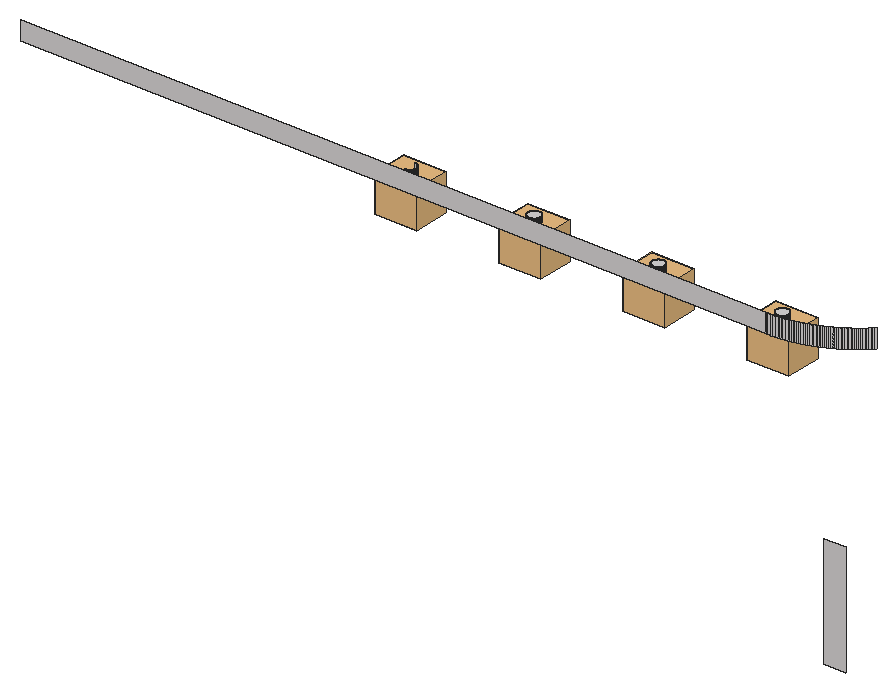
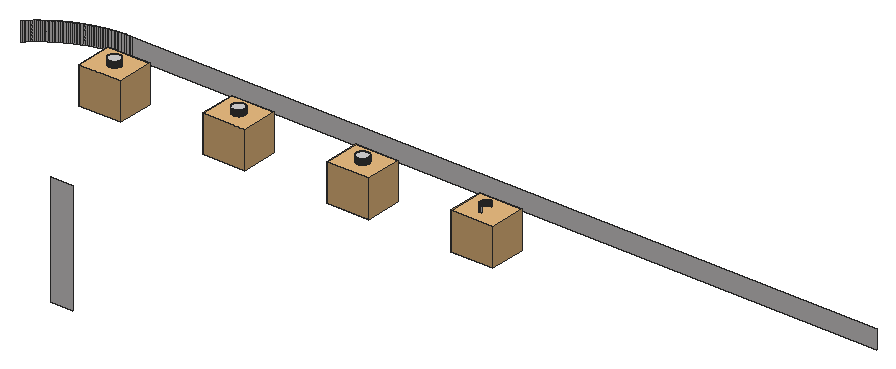
# SketchUp Ruby script. Lengths in inches.
U = 1.inch
M = Sketchup.active_model
def pt(a) = Geom::Point3d.new(a.map { |v| v * U })
def face(e, loops, mat)
  f = e.add_face(loops[0].map { |a| pt(a) })
  loops[1..].each { |l| e.add_face(l.map { |a| pt(a) }).erase! }
  f.material = f.back_material = mat if mat
  f
end
# faces: each face lists its corners as indices into pts; further lists are holes
def faces(e, pts, list, mat = nil) = list.each { |f| face(e, (f[0].is_a?(Array) ? f : [f]).map { |l| l.map { |i| pts[i] } }, mat) }
# xy, xz, yz: faces in a plane at the given z, y or x. An outline is a flat list of corners, or four numbers for a rectangle; further outlines are holes
def ring(l) = l.size == 4 ? [[l[0], l[1]], [l[2], l[1]], [l[2], l[3]], [l[0], l[3]]] : l.each_slice(2).to_a
def flat(e, list, mat, &to3) = list.each { |f| face(e, (f[0].is_a?(Array) ? f : [f]).map { |l| ring(l).map { |u, v| to3.(u, v) } }, mat) }
def xy(e, z, list, mat = nil) = flat(e, list, mat) { |x, y| [x, y, z] }
def xz(e, y, list, mat = nil) = flat(e, list, mat) { |x, z| [x, y, z] }
def yz(e, x, list, mat = nil) = flat(e, list, mat) { |y, z| [x, y, z] }
def lines(e, pts, list) = list.each { |a, b| e.add_line(pt(pts[a]), pt(pts[b])) }
# prism: a flat outline (further loops are holes) pulled along v
def prism(e, loops, v, mat = nil)
  f = face(e, loops, mat); d = Geom::Vector3d.new(v.map { |x| x * U })
  f.pushpull(f.normal.samedirection?(d) ? d.length : -d.length)
end
def box(e, o, s, mat = nil) = prism(e, [[o, [o[0] + s[0], o[1], o[2]], [o[0] + s[0], o[1] + s[1], o[2]], [o[0], o[1] + s[1], o[2]]]], [0, 0, s[2]], mat)
def at(x, y, z, deg = 0) = Geom::Transformation.translation(pt([x, y, z])) * Geom::Transformation.rotation(ORIGIN, Z_AXIS, deg.degrees)
def axes(o, x, y, z) = Geom::Transformation.new([*x, 0, *y, 0, *z, 0, *pt(o).to_a, 1])
def part(name) = M.definitions.add(name)
# library, detail: a bought-in or finely detailed component or shape, given as its bounding box
def library(name, o, s) = part(name).tap { |d| box(d.entities, o, s) }
def detail(e, o, s) = box(e.add_group.entities, o, s)
def put(e, d, t, mat = nil) = e.add_instance(d, t).tap { |i| i.material = mat if mat }
def group(e, t, mat = nil) = e.add_group.tap { |g| g.transformation = t; g.material = mat if mat }.entities
root = M.entities
M.materials.add("[Quartz Light Brown]").color = [215, 212, 212]
c1 = library("3",[-5.26,-4.28,-11.86],[13.52,11.56,11.86])
xy(root,483,[[384.27,287.7,384.11,287.71,383.81,287.77,383.66,287.82,383.51,287.88,383.37,287.95,383.24,288.03,383.11,288.12,382.99,288.22,382.875,288.33,382.77,288.45,382.68,288.58,382.6,288.71,382.52,288.85,382.46,288.99,382.41,289.14,382.375,289.29,382.35,289.45,382.34,289.61,382.33,289.76,382.37,290.08,382.4,290.23,382.45,290.38,382.51,290.52,382.58,290.66,382.66,290.8,382.75,290.93,382.85,291.05,382.96,291.16,383.08,291.26,383.21,291.35,383.34,291.4375,383.48,291.51,383.625,291.57,383.77,291.62,383.93,291.66,384.08,291.69,384.24,291.7,384.4,291.7,384.55,291.6875,384.71,291.67,384.86,291.63,385.01,291.58,385.16,291.52,385.3,291.45,385.43,291.37,385.56,291.28,385.68,291.18,385.79,291.07,385.99,290.83,386.07,290.69,386.14,290.55,386.2,290.41,386.25,290.26,386.29,290.11,386.32,289.95,386.33,289.8,386.33,289.64,386.32,289.48,386.3,289.33,386.26,289.17,386.22,289.02,386.16,288.88,386.09,288.74,386.01,288.6,385.91,288.48,385.8125,288.36,385.7,288.24,385.58,288.14,385.46,288.05,385.32,287.96,385.19,287.89,385.04,287.83,384.89,287.78,384.74,287.74,384.58,287.72,384.43,287.7],[424.1,287.7,423.95,287.71,423.79,287.74,423.64,287.77,423.49,287.82,423.34,287.88,423.2,287.95,423.07,288.03,422.94,288.12,422.82,288.22,422.71,288.33,422.61,288.45,422.51,288.58,422.43,288.71,422.36,288.85,422.3,288.99,422.25,289.14,422.21,289.29,422.18,289.45,422.17,289.61,422.17,289.76,422.18,289.92,422.2,290.08,422.28,290.38,422.34,290.52,422.41,290.66,422.49,290.8,422.59,290.93,422.6875,291.05,422.8,291.16,422.92,291.26,423.04,291.35,423.18,291.4375,423.31,291.51,423.46,291.57,423.61,291.62,423.76,291.66,423.92,291.69,424.07,291.7,424.23,291.7,424.39,291.6875,424.54,291.67,424.69,291.63,424.84,291.58,424.99,291.52,425.13,291.45,425.26,291.37,425.39,291.28,425.51,291.18,425.625,291.07,425.73,290.95,425.82,290.83,425.98,290.55,426.04,290.41,426.09,290.26,426.125,290.11,426.15,289.95,426.16,289.8,426.17,289.64,426.15,289.48,426.13,289.33,426.1,289.17,426.05,289.02,425.99,288.88,425.92,288.74,425.84,288.6,425.75,288.48,425.65,288.36,425.54,288.24,425.42,288.14,425.16,287.96,425.02,287.89,424.875,287.83,424.73,287.78,424.57,287.74,424.42,287.72,424.26,287.7],[463.9375,287.7,463.78,287.71,463.47,287.77,463.32,287.82,463.18,287.88,463.04,287.95,462.9,288.03,462.77,288.12,462.65,288.22,462.54,288.33,462.44,288.45,462.26,288.71,462.19,288.85,462.13,288.99,462.08,289.14,462.04,289.29,462,289.61,462,289.76,462.01,289.92,462.04,290.08,462.07,290.23,462.12,290.38,462.18,290.52,462.25,290.66,462.33,290.8,462.42,290.93,462.52,291.05,462.63,291.16,462.75,291.26,462.875,291.35,463.01,291.4375,463.15,291.51,463.29,291.57,463.44,291.62,463.59,291.66,463.75,291.69,463.91,291.7,464.0625,291.7,464.22,291.6875,464.375,291.67,464.53,291.63,464.68,291.58,464.82,291.52,464.96,291.45,465.1,291.37,465.23,291.28,465.35,291.18,465.46,291.07,465.56,290.95,465.65,290.83,465.74,290.69,465.81,290.55,465.87,290.41,465.92,290.26,465.96,290.11,465.98,289.95,466,289.8,466,289.64,465.99,289.48,465.96,289.33,465.93,289.17,465.88,289.02,465.82,288.88,465.75,288.74,465.67,288.6,465.58,288.48,465.48,288.36,465.37,288.24,465.25,288.14,465.125,288.05,464.99,287.96,464.85,287.89,464.71,287.83,464.56,287.78,464.41,287.74,464.09,287.7]],"[Quartz Light Brown]")
xz(root,276.5,[[488,396,495,432]],"[Quartz Light Brown]")
xz(root,282.7,[[225,480,464,486],[464,480,464.5,486]],"[Quartz Light Brown]")
xz(root,287.7,[[344.4375,480,344.59,483],[384.27,480,384.43,483],[424.1,480,424.26,483],[463.9375,480,464.09,483]],"[Quartz Light Brown]")
xz(root,291.7,[[384.24,480,384.4,483],[424.07,480,424.23,483],[463.91,480,464.0625,483]],"[Quartz Light Brown]")
yz(root,346.5,[[289.64,480,289.8,483]],"[Quartz Light Brown]")
yz(root,386.33,[[289.64,480,289.8,483]],"[Quartz Light Brown]")
yz(root,422.17,[[289.61,480,289.76,483]],"[Quartz Light Brown]")
yz(root,462,[[289.61,480,289.76,483]],"[Quartz Light Brown]")
yz(root,466,[[289.64,480,289.8,483]],"[Quartz Light Brown]")
p = [[464.5,282.7,480],[464.99,282.71,480],[464.99,282.71,486],[464.5,282.7,486],[465.49,282.73,480],[465.49,282.73,486],
  [465.99,282.75,480],[465.99,282.75,486],[466.49,282.78,480],[466.49,282.78,486],[466.98,282.82,480],[466.98,282.82,486],
  [467.48,282.86,480],[467.48,282.86,486],[467.97,282.91,480],[467.97,282.91,486],[468.47,282.96,480],[468.47,282.96,486],
  [468.96,283.03,480],[468.96,283.03,486],[469.45,283.09,480],[469.45,283.09,486],[469.94,283.17,480],[469.94,283.17,486],
  [470.44,283.25,480],[470.44,283.25,486],[470.92,283.34,480],[470.92,283.34,486],[471.41,283.43,480],[471.41,283.43,486],
  [471.9,283.53,480],[471.9,283.53,486],[472.39,283.64,480],[472.39,283.64,486],[472.87,283.75,480],[472.87,283.75,486],
  [473.35,283.87,480],[473.35,283.87,486],[473.84,284,480],[473.84,284,486],[474.31,284.13,480],[474.31,284.13,486],
  [474.79,284.27,480],[474.79,284.27,486],[475.27,284.41,480],[475.27,284.41,486],[475.74,284.5625,480],[475.74,284.5625,486],
  [476.21,284.72,480],[476.21,284.72,486],[476.68,284.88,480],[476.68,284.88,486],[477.15,285.05,480],[477.15,285.05,486],
  [477.62,285.22,480],[477.62,285.22,486],[478.08,285.41,480],[478.08,285.41,486],[478.54,285.59,480],[478.54,285.59,486],
  [479,285.79,480],[479,285.79,486],[479.46,285.99,480],[479.46,285.99,486],[479.91,286.19,480],[479.91,286.19,486],
  [480.36,286.4,480],[480.36,286.4,486],[480.81,286.62,480],[480.81,286.62,486],[481.25,286.84,480],[481.25,286.84,486],
  [481.69,287.07,480],[481.69,287.07,486],[482.13,287.31,480],[482.13,287.31,486],[482.57,287.55,480],[482.57,287.55,486],
  [483,287.79,480],[483,287.79,486],[344.75,287.72,480],[344.59,287.7,480],[344.59,287.7,483],[344.75,287.72,483],
  [344.91,287.74,480],[344.91,287.74,483],[345.06,287.78,480],[345.06,287.78,483],[383.96,287.74,480],[383.81,287.77,480],
  [383.81,287.77,483],[383.96,287.74,483],[384.11,287.71,480],[384.11,287.71,483],[384.27,287.7,480],[384.27,287.7,483],
  [384.58,287.72,480],[384.43,287.7,480],[384.43,287.7,483],[384.58,287.72,483],[384.74,287.74,480],[384.74,287.74,483],
  [384.89,287.78,480],[384.89,287.78,483],[423.79,287.74,480],[423.64,287.77,480],[423.64,287.77,483],[423.79,287.74,483],
  [423.95,287.71,480],[423.95,287.71,483],[424.1,287.7,480],[424.1,287.7,483],[424.42,287.72,480],[424.26,287.7,480],
  [424.26,287.7,483],[424.42,287.72,483],[424.57,287.74,480],[424.57,287.74,483],[424.73,287.78,480],[424.73,287.78,483],
  [463.625,287.74,480],[463.47,287.77,480],[463.47,287.77,483],[463.625,287.74,483],[463.78,287.71,480],[463.78,287.71,483],
  [463.9375,287.7,480],[463.9375,287.7,483],[464.25,287.72,480],[464.09,287.7,480],[464.09,287.7,483],[464.25,287.72,483],
  [464.41,287.74,480],[464.41,287.74,483],[464.56,287.78,480],[464.56,287.78,483],[345.21,287.83,480],[345.21,287.83,483],
  [345.35,287.89,480],[345.35,287.89,483],[383.66,287.82,480],[383.51,287.88,480],[383.51,287.88,483],[383.66,287.82,483],
  [385.04,287.83,480],[385.04,287.83,483],[385.19,287.89,480],[385.19,287.89,483],[423.49,287.82,480],[423.34,287.88,480],
  [423.34,287.88,483],[423.49,287.82,483],[424.875,287.83,480],[424.875,287.83,483],[425.02,287.89,480],[425.02,287.89,483],
  [463.32,287.82,480],[463.18,287.88,480],[463.18,287.88,483],[463.32,287.82,483],[464.71,287.83,480],[464.71,287.83,483],
  [464.85,287.89,480],[464.85,287.89,483],[483.43,288.04,480],[483.43,288.04,486],[345.49,287.96,480],[345.49,287.96,483],
  [383.37,287.95,480],[383.24,288.03,480],[383.24,288.03,483],[383.37,287.95,483],[385.32,287.96,480],[385.32,287.96,483],
  [423.2,287.95,480],[423.07,288.03,480],[423.07,288.03,483],[423.2,287.95,483],[425.16,287.96,480],[425.16,287.96,483],
  [463.04,287.95,480],[462.9,288.03,480],[462.9,288.03,483],[463.04,287.95,483],[464.99,287.96,480],[464.99,287.96,483],
  [345.625,288.05,480],[345.625,288.05,483],[345.75,288.14,480],[345.75,288.14,483],[383.11,288.12,480],[383.11,288.12,483],
  [385.46,288.05,480],[385.46,288.05,483],[385.58,288.14,480],[385.58,288.14,483],[422.94,288.12,480],[422.94,288.12,483],
  [425.29,288.05,480],[425.29,288.05,483],[425.42,288.14,480],[425.42,288.14,483],[462.77,288.12,480],[462.77,288.12,483],
  [465.125,288.05,480],[465.125,288.05,483],[465.25,288.14,480],[465.25,288.14,483],[483.85,288.3,480],[483.85,288.3,486],
  [345.87,288.24,480],[345.87,288.24,483],[382.99,288.22,480],[382.99,288.22,483],[385.7,288.24,480],[385.7,288.24,483],
  [422.82,288.22,480],[422.82,288.22,483],[425.54,288.24,480],[425.54,288.24,483],[462.65,288.22,480],[462.65,288.22,483],
  [465.37,288.24,480],[465.37,288.24,483],[345.98,288.36,480],[345.98,288.36,483],[382.875,288.33,480],[382.875,288.33,483],
  [385.8125,288.36,480],[385.8125,288.36,483],[422.71,288.33,480],[422.71,288.33,483],[425.65,288.36,480],[425.65,288.36,483],
  [462.54,288.33,480],[462.54,288.33,483],[465.48,288.36,480],[465.48,288.36,483],[382.77,288.45,480],[382.77,288.45,483],
  [422.61,288.45,480],[422.61,288.45,483],[462.44,288.45,480],[462.44,288.45,483],[484.28,288.5625,480],[484.28,288.5625,486],
  [346.08,288.48,480],[346.08,288.48,483],[385.91,288.48,480],[385.91,288.48,483],[425.75,288.48,480],[425.75,288.48,483],
  [465.58,288.48,480],[465.58,288.48,483],[346.17,288.6,480],[346.17,288.6,483],[382.68,288.58,480],[382.68,288.58,483],
  [386.01,288.6,480],[386.01,288.6,483],[422.51,288.58,480],[422.51,288.58,483],[425.84,288.6,480],[425.84,288.6,483],
  [462.35,288.58,480],[462.35,288.58,483],[465.67,288.6,480],[465.67,288.6,483],[346.25,288.74,480],[346.25,288.74,483],
  [382.6,288.71,480],[382.6,288.71,483],[386.09,288.74,480],[386.09,288.74,483],[422.43,288.71,480],[422.43,288.71,483],
  [425.92,288.74,480],[425.92,288.74,483],[462.26,288.71,480],[462.26,288.71,483],[465.75,288.74,480],[465.75,288.74,483],
  [484.7,288.83,480],[484.7,288.83,486],[346.32,288.88,480],[346.32,288.88,483],[382.52,288.85,480],[382.52,288.85,483],
  [386.16,288.88,480],[386.16,288.88,483],[422.36,288.85,480],[422.36,288.85,483],[425.99,288.88,480],[425.99,288.88,483],
  [462.19,288.85,480],[462.19,288.85,483],[465.82,288.88,480],[465.82,288.88,483],[382.46,288.99,480],[382.46,288.99,483],
  [422.3,288.99,480],[422.3,288.99,483],[462.13,288.99,480],[462.13,288.99,483],[485.11,289.11,480],[485.11,289.11,486],
  [346.38,289.02,480],[346.38,289.02,483],[386.22,289.02,480],[386.22,289.02,483],[426.05,289.02,480],[426.05,289.02,483],
  [465.88,289.02,480],[465.88,289.02,483],[346.43,289.17,480],[346.43,289.17,483],[382.41,289.14,480],[382.41,289.14,483],
  [386.26,289.17,480],[386.26,289.17,483],[422.25,289.14,480],[422.25,289.14,483],[426.1,289.17,480],[426.1,289.17,483],
  [462.08,289.14,480],[462.08,289.14,483],[465.93,289.17,480],[465.93,289.17,483],[382.375,289.29,480],[382.375,289.29,483],
  [422.21,289.29,480],[422.21,289.29,483],[462.04,289.29,480],[462.04,289.29,483],[485.52,289.38,480],[485.52,289.38,486],
  [346.46,289.33,480],[346.46,289.33,483],[386.3,289.33,480],[386.3,289.33,483],[426.13,289.33,480],[426.13,289.33,483],
  [465.96,289.33,480],[465.96,289.33,483],[346.49,289.48,480],[346.49,289.48,483],[382.35,289.45,480],[382.35,289.45,483],
  [386.32,289.48,480],[386.32,289.48,483],[422.18,289.45,480],[422.18,289.45,483],[426.15,289.48,480],[426.15,289.48,483],
  [462.02,289.45,480],[462.02,289.45,483],[465.99,289.48,480],[465.99,289.48,483],[382.34,289.61,480],[382.34,289.61,483],
  [422.17,289.61,480],[422.17,289.61,483],[462,289.61,480],[462,289.61,483],[485.93,289.67,480],[485.93,289.67,486],
  [346.5,289.64,480],[346.5,289.64,483],[386.33,289.64,480],[386.33,289.64,483],[426.17,289.64,480],[426.17,289.64,483],
  [466,289.64,480],[466,289.64,483],[382.33,289.76,480],[382.33,289.76,483],[426.16,289.8,480],[426.16,289.8,483],
  [486.34,289.96,480],[486.34,289.96,486],[346.48,289.95,480],[346.5,289.8,480],[346.5,289.8,483],[346.48,289.95,483],
  [382.35,289.92,480],[382.35,289.92,483],[386.32,289.95,480],[386.33,289.8,480],[386.33,289.8,483],[386.32,289.95,483],
  [422.17,289.76,480],[422.18,289.92,480],[422.18,289.92,483],[422.17,289.76,483],[426.15,289.95,480],[426.15,289.95,483],
  [462,289.76,480],[462.01,289.92,480],[462.01,289.92,483],[462,289.76,483],[465.98,289.95,480],[466,289.8,480],
  [466,289.8,483],[465.98,289.95,483],[382.37,290.08,480],[382.37,290.08,483],[422.2,290.08,480],[422.2,290.08,483],
  [462.04,290.08,480],[462.04,290.08,483],[346.46,290.11,480],[346.46,290.11,483],[386.29,290.11,480],[386.29,290.11,483],
  [426.125,290.11,480],[426.125,290.11,483],[465.96,290.11,480],[465.96,290.11,483],[486.74,290.25,480],[486.74,290.25,486],
  [346.42,290.26,480],[346.42,290.26,483],[382.4,290.23,480],[382.4,290.23,483],[386.25,290.26,480],[386.25,290.26,483],
  [422.24,290.23,480],[422.24,290.23,483],[426.09,290.26,480],[426.09,290.26,483],[462.07,290.23,480],[462.07,290.23,483],
  [465.92,290.26,480],[465.92,290.26,483],[382.45,290.38,480],[382.45,290.38,483],[422.28,290.38,480],[422.28,290.38,483],
  [462.12,290.38,480],[462.12,290.38,483],[346.37,290.41,480],[346.37,290.41,483],[386.2,290.41,480],[386.2,290.41,483],
  [426.04,290.41,480],[426.04,290.41,483],[465.87,290.41,480],[465.87,290.41,483],[487.13,290.55,480],[487.13,290.55,486],
  [346.31,290.55,480],[346.31,290.55,483],[382.51,290.52,480],[382.51,290.52,483],[386.14,290.55,480],[386.14,290.55,483],
  [422.34,290.52,480],[422.34,290.52,483],[425.98,290.55,480],[425.98,290.55,483],[462.18,290.52,480],[462.18,290.52,483],
  [465.81,290.55,480],[465.81,290.55,483],[382.58,290.66,480],[382.58,290.66,483],[422.41,290.66,480],[422.41,290.66,483],
  [462.25,290.66,480],[462.25,290.66,483],[346.24,290.69,480],[346.24,290.69,483],[386.07,290.69,480],[386.07,290.69,483],
  [425.9,290.69,480],[425.9,290.69,483],[465.74,290.69,480],[465.74,290.69,483],[487.53,290.86,480],[487.53,290.86,486],
  [346.15,290.83,480],[346.15,290.83,483],[382.66,290.8,480],[382.66,290.8,483],[385.99,290.83,480],[385.99,290.83,483],
  [422.49,290.8,480],[422.49,290.8,483],[425.82,290.83,480],[425.82,290.83,483],[462.33,290.8,480],[462.33,290.8,483],
  [465.65,290.83,480],[465.65,290.83,483],[346.06,290.95,480],[346.06,290.95,483],[382.75,290.93,480],[382.75,290.93,483],
  [385.89,290.95,480],[385.89,290.95,483],[422.59,290.93,480],[422.59,290.93,483],[425.73,290.95,480],[425.73,290.95,483],
  [462.42,290.93,480],[462.42,290.93,483],[465.56,290.95,480],[465.56,290.95,483],[382.85,291.05,480],[382.85,291.05,483],
  [422.6875,291.05,480],[422.6875,291.05,483],[462.52,291.05,480],[462.52,291.05,483],[487.91,291.17,480],[487.91,291.17,486],
  [345.96,291.07,480],[345.96,291.07,483],[382.96,291.16,480],[382.96,291.16,483],[385.79,291.07,480],[385.79,291.07,483],
  [422.8,291.16,480],[422.8,291.16,483],[425.625,291.07,480],[425.625,291.07,483],[462.63,291.16,480],[462.63,291.16,483],
  [465.46,291.07,480],[465.46,291.07,483],[345.85,291.18,480],[345.85,291.18,483],[385.68,291.18,480],[385.68,291.18,483],
  [425.51,291.18,480],[425.51,291.18,483],[465.35,291.18,480],[465.35,291.18,483],[345.73,291.28,480],[345.73,291.28,483],
  [383.08,291.26,480],[383.08,291.26,483],[385.56,291.28,480],[385.56,291.28,483],[422.92,291.26,480],[422.92,291.26,483],
  [425.39,291.28,480],[425.39,291.28,483],[462.75,291.26,480],[462.75,291.26,483],[465.23,291.28,480],[465.23,291.28,483],
  [488.3,291.49,480],[488.3,291.49,486],[345.6,291.37,480],[345.6,291.37,483],[383.21,291.35,480],[383.21,291.35,483],
  [385.43,291.37,480],[385.43,291.37,483],[423.04,291.35,480],[423.04,291.35,483],[425.26,291.37,480],[425.26,291.37,483],
  [462.875,291.35,480],[462.875,291.35,483],[465.1,291.37,480],[465.1,291.37,483],[345.46,291.45,480],[345.46,291.45,483],
  [383.34,291.4375,480],[383.34,291.4375,483],[383.48,291.51,480],[383.48,291.51,483],[385.3,291.45,480],[385.3,291.45,483],
  [423.18,291.4375,480],[423.18,291.4375,483],[423.31,291.51,480],[423.31,291.51,483],[425.13,291.45,480],[425.13,291.45,483],
  [463.01,291.4375,480],[463.01,291.4375,483],[463.15,291.51,480],[463.15,291.51,483],[464.96,291.45,480],[464.96,291.45,483],
  [345.18,291.58,480],[345.32,291.52,480],[345.32,291.52,483],[345.18,291.58,483],[383.625,291.57,480],[383.625,291.57,483],
  [385.01,291.58,480],[385.16,291.52,480],[385.16,291.52,483],[385.01,291.58,483],[423.46,291.57,480],[423.46,291.57,483],
  [424.84,291.58,480],[424.99,291.52,480],[424.99,291.52,483],[424.84,291.58,483],[463.29,291.57,480],[463.29,291.57,483],
  [464.68,291.58,480],[464.82,291.52,480],[464.82,291.52,483],[464.68,291.58,483],[488.68,291.81,480],[488.68,291.81,486],
  [344.875,291.67,480],[345.03,291.63,480],[345.03,291.63,483],[344.875,291.67,483],[383.77,291.62,480],[383.77,291.62,483],
  [383.93,291.66,480],[383.93,291.66,483],[384.71,291.67,480],[384.86,291.63,480],[384.86,291.63,483],[384.71,291.67,483],
  [423.61,291.62,480],[423.61,291.62,483],[423.76,291.66,480],[423.76,291.66,483],[424.54,291.67,480],[424.69,291.63,480],
  [424.69,291.63,483],[424.54,291.67,483],[463.44,291.62,480],[463.44,291.62,483],[463.59,291.66,480],[463.59,291.66,483],
  [464.375,291.67,480],[464.53,291.63,480],[464.53,291.63,483],[464.375,291.67,483],[344.5625,291.7,480],[344.72,291.6875,480],
  [344.72,291.6875,483],[344.5625,291.7,483],[384.08,291.69,480],[384.08,291.69,483],[384.24,291.7,480],[384.24,291.7,483],
  [384.4,291.7,480],[384.55,291.6875,480],[384.55,291.6875,483],[384.4,291.7,483],[423.92,291.69,480],[423.92,291.69,483],
  [424.07,291.7,480],[424.07,291.7,483],[424.23,291.7,480],[424.39,291.6875,480],[424.39,291.6875,483],[424.23,291.7,483],
  [463.75,291.69,480],[463.75,291.69,483],[463.91,291.7,480],[463.91,291.7,483],[464.0625,291.7,480],[464.22,291.6875,480],
  [464.22,291.6875,483],[464.0625,291.7,483],[489.06,292.13,480],[489.06,292.13,486],[489.43,292.46,480],[489.43,292.46,486],
  [489.79,292.8,480],[489.79,292.8,486],[490.16,293.14,480],[490.16,293.14,486],[490.52,293.48,480],[490.52,293.48,486],
  [490.87,293.83,480],[490.87,293.83,486]]
faces(root,p,[[0,1,2,3],[1,4,5,2],[4,6,7,5],[6,8,9,7],[8,10,11,9],[10,12,13,11],[12,14,15,13],[14,16,17,15],
  [16,18,19,17],[18,20,21,19],[20,22,23,21],[22,24,25,23],[24,26,27,25],[26,28,29,27],[28,30,31,29],[30,32,33,31],
  [32,34,35,33],[34,36,37,35],[36,38,39,37],[38,40,41,39],[40,42,43,41],[42,44,45,43],[44,46,47,45],[46,48,49,47],
  [48,50,51,49],[50,52,53,51],[52,54,55,53],[54,56,57,55],[56,58,59,57],[58,60,61,59],[60,62,63,61],[62,64,65,63],
  [64,66,67,65],[66,68,69,67],[68,70,71,69],[70,72,73,71],[72,74,75,73],[74,76,77,75],[76,78,79,77],[80,81,82,83],
  [84,80,83,85],[86,84,85,87],[88,89,90,91],[92,88,91,93],[94,92,93,95],[96,97,98,99],[100,96,99,101],[102,100,101,103],
  [104,105,106,107],[108,104,107,109],[110,108,109,111],[112,113,114,115],[116,112,115,117],[118,116,117,119],[120,121,122,123],[124,120,123,125],
  [126,124,125,127],[128,129,130,131],[132,128,131,133],[134,132,133,135],[136,86,87,137],[138,136,137,139],[140,141,142,143],[89,140,143,90],
  [144,102,103,145],[146,144,145,147],[148,149,150,151],[105,148,151,106],[152,118,119,153],[154,152,153,155],[156,157,158,159],[121,156,159,122],
  [160,134,135,161],[162,160,161,163],[78,164,165,79],[166,138,139,167],[168,169,170,171],[141,168,171,142],[172,146,147,173],[174,175,176,177],
  [149,174,177,150],[178,154,155,179],[180,181,182,183],[157,180,183,158],[184,162,163,185],[186,166,167,187],[188,186,187,189],[169,190,191,170],
  [192,172,173,193],[194,192,193,195],[175,196,197,176],[198,178,179,199],[200,198,199,201],[181,202,203,182],[204,184,185,205],[206,204,205,207],
  [164,208,209,165],[210,188,189,211],[190,212,213,191],[214,194,195,215],[196,216,217,197],[218,200,201,219],[202,220,221,203],[222,206,207,223],
  [224,210,211,225],[212,226,227,213],[228,214,215,229],[216,230,231,217],[232,218,219,233],[220,234,235,221],[236,222,223,237],[226,238,239,227],
  [230,240,241,231],[234,242,243,235],[208,244,245,209],[246,224,225,247],[248,228,229,249],[250,232,233,251],[252,236,237,253],[254,246,247,255],
  [238,256,257,239],[258,248,249,259],[240,260,261,241],[262,250,251,263],[242,264,265,243],[266,252,253,267],[268,254,255,269],[256,270,271,257],
  [272,258,259,273],[260,274,275,261],[276,262,263,277],[264,278,279,265],[280,266,267,281],[244,282,283,245],[284,268,269,285],[270,286,287,271],
  [288,272,273,289],[274,290,291,275],[292,276,277,293],[278,294,295,279],[296,280,281,297],[286,298,299,287],[290,300,301,291],[294,302,303,295],
  [282,304,305,283],[306,284,285,307],[308,288,289,309],[310,292,293,311],[312,296,297,313],[314,306,307,315],[298,316,317,299],[318,308,309,319],
  [300,320,321,301],[322,310,311,323],[302,324,325,303],[326,312,313,327],[316,328,329,317],[320,330,331,321],[324,332,333,325],[304,334,335,305],
  [336,314,315,337],[338,318,319,339],[340,322,323,341],[342,326,327,343],[344,336,337,345],[328,346,347,329],[348,338,339,349],[330,350,351,331],
  [352,340,341,353],[332,354,355,333],[356,342,343,357],[346,358,359,347],[350,360,361,351],[354,362,363,355],[334,364,365,335],[366,344,345,367],
  [368,348,349,369],[370,352,353,371],[372,356,357,373],[358,374,375,359],[376,370,371,377],[364,378,379,365],[380,381,382,383],[374,384,385,375],
  [386,387,388,389],[390,391,392,393],[394,376,377,395],[396,397,398,399],[400,401,402,403],[384,404,405,385],[391,406,407,392],[397,408,409,398],
  [410,380,383,411],[412,386,389,413],[414,394,395,415],[416,400,403,417],[378,418,419,379],[420,410,411,421],[404,422,423,405],[424,412,413,425],
  [406,426,427,407],[428,414,415,429],[408,430,431,409],[432,416,417,433],[422,434,435,423],[426,436,437,427],[430,438,439,431],[440,420,421,441],
  [442,424,425,443],[444,428,429,445],[446,432,433,447],[418,448,449,419],[450,440,441,451],[434,452,453,435],[454,442,443,455],[436,456,457,437],
  [458,444,445,459],[438,460,461,439],[462,446,447,463],[452,464,465,453],[456,466,467,457],[460,468,469,461],[470,450,451,471],[472,454,455,473],
  [474,458,459,475],[476,462,463,477],[448,478,479,449],[480,470,471,481],[464,482,483,465],[484,472,473,485],[466,486,487,467],[488,474,475,489],
  [468,490,491,469],[492,476,477,493],[494,480,481,495],[482,496,497,483],[498,484,485,499],[486,500,501,487],[502,488,489,503],[490,504,505,491],
  [506,492,493,507],[496,508,509,497],[500,510,511,501],[504,512,513,505],[478,514,515,479],[516,494,495,517],[508,518,519,509],[520,498,499,521],
  [510,522,523,511],[524,502,503,525],[512,526,527,513],[528,506,507,529],[530,516,517,531],[532,520,521,533],[534,524,525,535],[536,528,529,537],
  [538,530,531,539],[518,540,541,519],[542,532,533,543],[522,544,545,523],[546,534,535,547],[526,548,549,527],[550,536,537,551],[514,552,553,515],
  [554,538,539,555],[540,556,557,541],[558,542,543,559],[544,560,561,545],[562,546,547,563],[548,564,565,549],[566,550,551,567],[568,554,555,569],
  [556,570,571,557],[570,572,573,571],[574,558,559,575],[560,576,577,561],[576,578,579,577],[580,562,563,581],[564,582,583,565],[582,584,585,583],
  [586,566,567,587],[588,589,590,591],[589,568,569,590],[572,592,593,573],[594,595,596,597],[595,574,575,596],[578,598,599,579],[600,601,602,603],
  [601,580,581,602],[584,604,605,585],[606,607,608,609],[607,586,587,608],[552,610,611,553],[612,613,614,615],[613,588,591,614],[592,616,617,593],
  [616,618,619,617],[620,621,622,623],[621,594,597,622],[598,624,625,599],[624,626,627,625],[628,629,630,631],[629,600,603,630],[604,632,633,605],
  [632,634,635,633],[636,637,638,639],[637,606,609,638],[640,641,642,643],[641,612,615,642],[618,644,645,619],[644,646,647,645],[648,649,650,651],
  [649,620,623,650],[626,652,653,627],[652,654,655,653],[656,657,658,659],[657,628,631,658],[634,660,661,635],[660,662,663,661],[664,665,666,667],
  [665,636,639,666],[610,668,669,611],[668,670,671,669],[670,672,673,671],[672,674,675,673],[674,676,677,675],[676,678,679,677]],"[Quartz Light Brown]")
put(root,c1,at(343,288.2,481.25),"[Quartz Light Brown]")
put(root,c1,at(382.83,288.2,481.25),"[Quartz Light Brown]")
put(root,c1,at(422.67,288.2,481.25),"[Quartz Light Brown]")
put(root,c1,at(462.5,288.2,481.25),"[Quartz Light Brown]")
